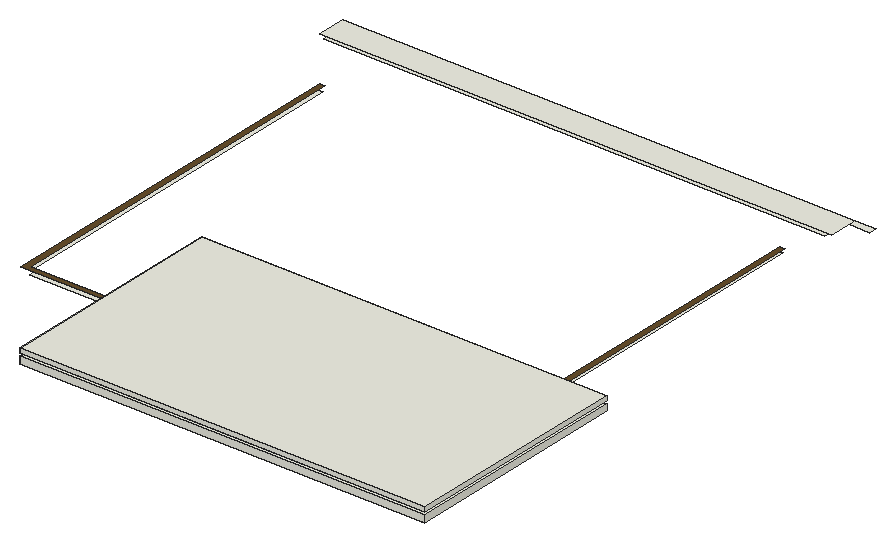
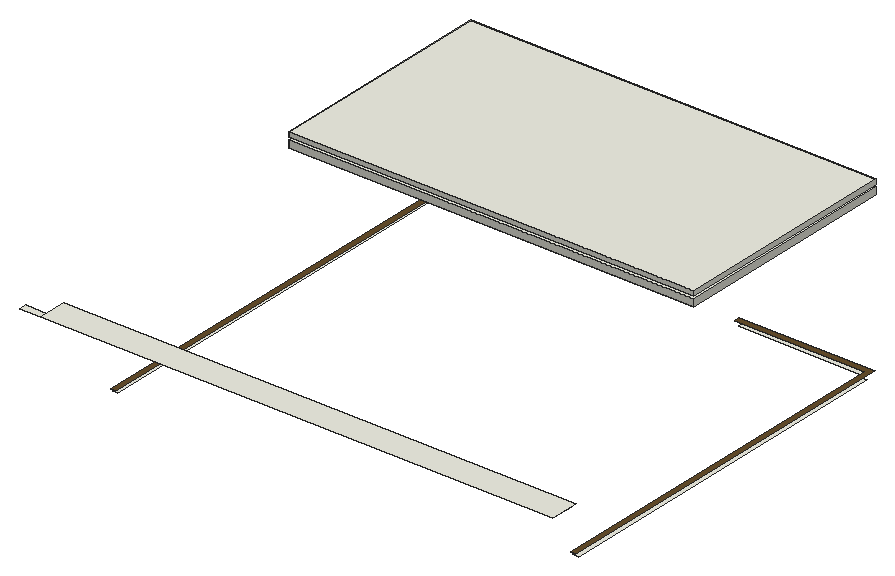
# SketchUp Ruby script. Lengths in inches.
U = 1.inch
M = Sketchup.active_model
def pt(a) = Geom::Point3d.new(a.map { |v| v * U })
def face(e, loops, mat)
  f = e.add_face(loops[0].map { |a| pt(a) })
  loops[1..].each { |l| e.add_face(l.map { |a| pt(a) }).erase! }
  f.material = f.back_material = mat if mat
  f
end
# faces: each face lists its corners as indices into pts; further lists are holes
def faces(e, pts, list, mat = nil) = list.each { |f| face(e, (f[0].is_a?(Array) ? f : [f]).map { |l| l.map { |i| pts[i] } }, mat) }
# xy, xz, yz: faces in a plane at the given z, y or x. An outline is a flat list of corners, or four numbers for a rectangle; further outlines are holes
def ring(l) = l.size == 4 ? [[l[0], l[1]], [l[2], l[1]], [l[2], l[3]], [l[0], l[3]]] : l.each_slice(2).to_a
def flat(e, list, mat, &to3) = list.each { |f| face(e, (f[0].is_a?(Array) ? f : [f]).map { |l| ring(l).map { |u, v| to3.(u, v) } }, mat) }
def xy(e, z, list, mat = nil) = flat(e, list, mat) { |x, y| [x, y, z] }
def xz(e, y, list, mat = nil) = flat(e, list, mat) { |x, z| [x, y, z] }
def yz(e, x, list, mat = nil) = flat(e, list, mat) { |y, z| [x, y, z] }
def lines(e, pts, list) = list.each { |a, b| e.add_line(pt(pts[a]), pt(pts[b])) }
# prism: a flat outline (further loops are holes) pulled along v
def prism(e, loops, v, mat = nil)
  f = face(e, loops, mat); d = Geom::Vector3d.new(v.map { |x| x * U })
  f.pushpull(f.normal.samedirection?(d) ? d.length : -d.length)
end
def box(e, o, s, mat = nil) = prism(e, [[o, [o[0] + s[0], o[1], o[2]], [o[0] + s[0], o[1] + s[1], o[2]], [o[0], o[1] + s[1], o[2]]]], [0, 0, s[2]], mat)
def at(x, y, z, deg = 0) = Geom::Transformation.translation(pt([x, y, z])) * Geom::Transformation.rotation(ORIGIN, Z_AXIS, deg.degrees)
def axes(o, x, y, z) = Geom::Transformation.new([*x, 0, *y, 0, *z, 0, *pt(o).to_a, 1])
def part(name) = M.definitions.add(name)
# library, detail: a bought-in or finely detailed component or shape, given as its bounding box
def library(name, o, s) = part(name).tap { |d| box(d.entities, o, s) }
def detail(e, o, s) = box(e.add_group.entities, o, s)
def put(e, d, t, mat = nil) = e.add_instance(d, t).tap { |i| i.material = mat if mat }
def group(e, t, mat = nil) = e.add_group.tap { |g| g.transformation = t; g.material = mat if mat }.entities
root = M.entities
M.materials.add("D01_Frost_White").color = [238, 238, 227]
M.materials.add("Wood_Veneer_15_1K").color = [103, 79, 44]
c1 = library("Sphere Light\#11",[-6.67,-6.67,-6.67],[13.34,13.34,13.34])
c2 = library("Sphere Light\#4",[-6.56,-6.56,-6.56],[13.12,13.12,13.12])
c3 = library("Sphere Light\#6",[-6.51,-6.51,-6.51],[13.02,13.02,13.02])
c4 = library("Sphere Light\#10",[-6.32,-6.32,-6.32],[12.64,12.64,12.64])
c5 = library("Sphere Light\#2",[-6.18,-6.18,-6.18],[12.36,12.36,12.36])
c6 = library("Sphere Light\#14",[-5.96,-5.96,-5.96],[11.92,11.92,11.92])
c7 = library("Sphere Light\#12",[-5.88,-5.88,-5.88],[11.76,11.76,11.76])
c8 = library("Sphere Light\#13",[-5.78,-5.78,-5.78],[11.56,11.56,11.56])
c9 = library("Sphere Light\#5",[-5.67,-5.67,-5.67],[11.34,11.34,11.34])
c10 = library("Sphere Light\#3",[-5.33,-5.33,-5.33],[10.66,10.66,10.66])
c11 = library("Sphere Light\#9",[-5.28,-5.28,-5.28],[10.56,10.56,10.56])
c12 = library("Sphere Light\#7",[-4.97,-4.97,-4.97],[9.94,9.94,9.94])
c13 = library("Sphere Light\#8",[-4.8125,-4.8125,-4.8125],[9.625,9.625,9.625])
xy(root,303,[[11.5,361,115,365.5],[4,368.5,8.5,673.01]],"D01_Frost_White")
xy(root,304,[[377.5,365.5,382,692]],"D01_Frost_White")
xy(root,306,[[4,361,118,361,118,365.5,8.5,365.5,8.5,676.01,4,676.01],[316,361,382,361,382,694,377.5,694,377.5,365.5,316,365.5]],"Wood_Veneer_15_1K")
xy(root,336,[[[118,217,460,409],[316,265,322,265,322,269,334,269,334,265,340,265,340,269,346,269,346,265,352,265,352,269,358,269,358,265,364,265,364,269,370,269,370,265,376,265,376,269,382,269,382,265,388,265,388,269,394,269,394,265,400,265,400,269,406,269,406,265,412,265,412,271,408,271,408,277,412,277,412,283,408,283,408,289,412,289,412,295,408,295,408,301,412,301,412,307,408,307,408,313,412,313,412,319,408,319,408,325,412,325,412,331,408,331,408,337,412,337,412,343,408,343,408,349,412,349,412,355,408,355,408,361,316,361,316,355,320,355,320,349,316,349,316,343,320,343,320,337,316,337,316,331,320,331,320,325,316,325,316,319,320,319,320,313,316,313,316,307,320,307,320,301,316,301,316,295,320,295,320,289,316,289,316,283,320,283,320,271,316,271],[142,373,166,385],[142,241,166,253],[448,271,449.55,271.2,451,271.8,452.24,272.76,453.2,274,453.8,275.45,454,277,453.8,278.55,453.2,280,452.24,281.24,451,282.2,449.55,282.8,448,283,446.45,282.8,445,282.2,443.76,281.24,442.8,280,442.2,278.55,442,277,442.2,275.45,442.8,274,443.76,272.76,445,271.8,446.45,271.2],[407,223,408.55,223.2,410,223.8,411.24,224.76,412.2,226,412.8,227.45,413,229,412.8,230.55,412.2,232,411.24,233.24,410,234.2,408.55,234.8,407,235,405.45,234.8,404,234.2,402.76,233.24,401.8,232,401.2,230.55,401,229,401.2,227.45,401.8,226,402.76,224.76,404,223.8,405.45,223.2],[448,307,449.55,307.2,451,307.8,452.24,308.76,453.2,310,453.8,311.45,454,313,453.8,314.55,453.2,316,452.24,317.24,451,318.2,449.55,318.8,448,319,446.45,318.8,445,318.2,443.76,317.24,442.8,316,442.2,314.55,442,313,442.2,311.45,442.8,310,443.76,308.76,445,307.8,446.45,307.2],[195,223,196.55,223.2,198,223.8,199.24,224.76,200.2,226,200.8,227.45,201,229,200.8,230.55,200.2,232,199.24,233.24,198,234.2,196.55,234.8,195,235,193.45,234.8,192,234.2,190.76,233.24,189.8,232,189.2,230.55,189,229,189.2,227.45,189.8,226,190.76,224.76,192,223.8,193.45,223.2],[248,223,249.55,223.2,251,223.8,252.24,224.76,253.2,226,253.8,227.45,254,229,253.8,230.55,253.2,232,252.24,233.24,251,234.2,249.55,234.8,248,235,246.45,234.8,245,234.2,243.76,233.24,242.8,232,242.2,230.55,242,229,242.2,227.45,242.8,226,243.76,224.76,245,223.8,246.45,223.2],[301,223,302.55,223.2,304,223.8,305.24,224.76,306.2,226,306.8,227.45,307,229,306.8,230.55,306.2,232,305.24,233.24,304,234.2,302.55,234.8,301,235,299.45,234.8,298,234.2,296.76,233.24,295.8,232,295.2,230.55,295,229,295.2,227.45,295.8,226,296.76,224.76,298,223.8,299.45,223.2],[354,223,355.55,223.2,357,223.8,358.24,224.76,359.2,226,359.8,227.45,360,229,359.8,230.55,359.2,232,358.24,233.24,357,234.2,355.55,234.8,354,235,352.45,234.8,351,234.2,349.76,233.24,348.8,232,348.2,230.55,348,229,348.2,227.45,348.8,226,349.76,224.76,351,223.8,352.45,223.2],[232,391,233.55,391.2,235,391.8,236.24,392.76,237.2,394,237.8,395.45,238,397,237.8,398.55,237.2,400,236.24,401.24,235,402.2,233.55,402.8,232,403,230.45,402.8,229,402.2,227.76,401.24,226.8,400,226.2,398.55,226,397,226.2,395.45,226.8,394,227.76,392.76,229,391.8,230.45,391.2],[403,391,404.55,391.2,406,391.8,407.24,392.76,408.2,394,408.8,395.45,409,397,408.8,398.55,408.2,400,407.24,401.24,406,402.2,404.55,402.8,403,403,401.45,402.8,400,402.2,398.76,401.24,397.8,400,397.2,398.55,397,397,397.2,395.45,397.8,394,398.76,392.76,400,391.8,401.45,391.2],[346,391,347.55,391.2,349,391.8,350.24,392.76,351.2,394,351.8,395.45,352,397,351.8,398.55,351.2,400,350.24,401.24,349,402.2,347.55,402.8,346,403,344.45,402.8,343,402.2,341.76,401.24,340.8,400,340.2,398.55,340,397,340.2,395.45,340.8,394,341.76,392.76,343,391.8,344.45,391.2],[289,391,290.55,391.2,292,391.8,293.24,392.76,294.2,394,294.8,395.45,295,397,294.8,398.55,294.2,400,293.24,401.24,292,402.2,290.55,402.8,289,403,287.45,402.8,286,402.2,284.76,401.24,283.8,400,283.2,398.55,283,397,283.2,395.45,283.8,394,284.76,392.76,286,391.8,287.45,391.2],[175,391,176.55,391.2,178,391.8,179.24,392.76,180.2,394,180.8,395.45,181,397,180.8,398.55,180.2,400,179.24,401.24,178,402.2,176.55,402.8,175,403,173.45,402.8,172,402.2,170.76,401.24,169.8,400,169.2,398.55,169,397,169.2,395.45,169.8,394,170.76,392.76,172,391.8,173.45,391.2],[448,343,449.55,343.2,451,343.8,452.24,344.76,453.2,346,453.8,347.45,454,349,453.8,350.55,453.2,352,452.24,353.24,451,354.2,449.55,354.8,448,355,446.45,354.8,445,354.2,443.76,353.24,442.8,352,442.2,350.55,442,349,442.2,347.45,442.8,346,443.76,344.76,445,343.8,446.45,343.2]],[316,265,322,265,322,269,334,269,334,265,340,265,340,269,346,269,346,265,352,265,352,269,358,269,358,265,364,265,364,269,370,269,370,265,376,265,376,269,382,269,382,265,388,265,388,269,394,269,394,265,400,265,400,269,406,269,406,265,412,265,412,271,316,271],[320,271,322,271,322,361,316,361,316,355,320,355,320,349,316,349,316,343,320,343,320,337,316,337,316,331,320,331,320,325,316,325,316,319,320,319,320,313,316,313,316,307,320,307,320,301,316,301,316,295,320,295,320,289,316,289,316,283,320,283],[322,271,406,355],[406,271,408,271,408,277,412,277,412,283,408,283,408,289,412,289,412,295,408,295,408,301,412,301,412,307,408,307,408,313,412,313,412,319,408,319,408,325,412,325,412,331,408,331,408,337,412,337,412,343,408,343,408,349,412,349,412,355,408,355,408,361,406,361],
  [322,355,406,361]],"D01_Frost_White")
xy(root,339,[[195,223,193.45,223.2,192,223.8,190.76,224.76,189.8,226,189.2,227.45,189,229,189.2,230.55,189.8,232,190.76,233.24,192,234.2,193.45,234.8,195,235,196.55,234.8,198,234.2,199.24,233.24,200.2,232,200.8,230.55,201,229,200.8,227.45,200.2,226,199.24,224.76,198,223.8,196.55,223.2],[248,223,246.45,223.2,245,223.8,243.76,224.76,242.8,226,242.2,227.45,242,229,242.2,230.55,242.8,232,243.76,233.24,245,234.2,246.45,234.8,248,235,249.55,234.8,251,234.2,252.24,233.24,253.2,232,253.8,230.55,254,229,253.8,227.45,253.2,226,252.24,224.76,251,223.8,249.55,223.2],[301,223,299.45,223.2,298,223.8,296.76,224.76,295.8,226,295.2,227.45,295,229,295.2,230.55,295.8,232,296.76,233.24,298,234.2,299.45,234.8,301,235,302.55,234.8,304,234.2,305.24,233.24,306.2,232,306.8,230.55,307,229,306.8,227.45,306.2,226,305.24,224.76,304,223.8,302.55,223.2],[354,223,352.45,223.2,351,223.8,349.76,224.76,348.8,226,348.2,227.45,348,229,348.2,230.55,348.8,232,349.76,233.24,351,234.2,352.45,234.8,354,235,355.55,234.8,357,234.2,358.24,233.24,359.2,232,359.8,230.55,360,229,359.8,227.45,359.2,226,358.24,224.76,357,223.8,355.55,223.2],[407,223,405.45,223.2,404,223.8,402.76,224.76,401.8,226,401.2,227.45,401,229,401.2,230.55,401.8,232,402.76,233.24,404,234.2,405.45,234.8,407,235,408.55,234.8,410,234.2,411.24,233.24,412.2,232,412.8,230.55,413,229,412.8,227.45,412.2,226,411.24,224.76,410,223.8,408.55,223.2],
  [448,271,446.45,271.2,445,271.8,443.76,272.76,442.8,274,442.2,275.45,442,277,442.2,278.55,442.8,280,443.76,281.24,445,282.2,446.45,282.8,448,283,449.55,282.8,451,282.2,452.24,281.24,453.2,280,453.8,278.55,454,277,453.8,275.45,453.2,274,452.24,272.76,451,271.8,449.55,271.2],[448,307,446.45,307.2,445,307.8,443.76,308.76,442.8,310,442.2,311.45,442,313,442.2,314.55,442.8,316,443.76,317.24,445,318.2,446.45,318.8,448,319,449.55,318.8,451,318.2,452.24,317.24,453.2,316,453.8,314.55,454,313,453.8,311.45,453.2,310,452.24,308.76,451,307.8,449.55,307.2],[448,343,446.45,343.2,445,343.8,443.76,344.76,442.8,346,442.2,347.45,442,349,442.2,350.55,442.8,352,443.76,353.24,445,354.2,446.45,354.8,448,355,449.55,354.8,451,354.2,452.24,353.24,453.2,352,453.8,350.55,454,349,453.8,347.45,453.2,346,452.24,344.76,451,343.8,449.55,343.2],[175,391,173.45,391.2,172,391.8,170.76,392.76,169.8,394,169.2,395.45,169,397,169.2,398.55,169.8,400,170.76,401.24,172,402.2,173.45,402.8,175,403,176.55,402.8,178,402.2,179.24,401.24,180.2,400,180.8,398.55,181,397,180.8,395.45,180.2,394,179.24,392.76,178,391.8,176.55,391.2],[232,391,230.45,391.2,229,391.8,227.76,392.76,226.8,394,226.2,395.45,226,397,226.2,398.55,226.8,400,227.76,401.24,229,402.2,230.45,402.8,232,403,233.55,402.8,235,402.2,236.24,401.24,237.2,400,237.8,398.55,238,397,237.8,395.45,237.2,394,236.24,392.76,235,391.8,233.55,391.2],
  [289,391,287.45,391.2,286,391.8,284.76,392.76,283.8,394,283.2,395.45,283,397,283.2,398.55,283.8,400,284.76,401.24,286,402.2,287.45,402.8,289,403,290.55,402.8,292,402.2,293.24,401.24,294.2,400,294.8,398.55,295,397,294.8,395.45,294.2,394,293.24,392.76,292,391.8,290.55,391.2],[346,391,344.45,391.2,343,391.8,341.76,392.76,340.8,394,340.2,395.45,340,397,340.2,398.55,340.8,400,341.76,401.24,343,402.2,344.45,402.8,346,403,347.55,402.8,349,402.2,350.24,401.24,351.2,400,351.8,398.55,352,397,351.8,395.45,351.2,394,350.24,392.76,349,391.8,347.55,391.2],[403,391,401.45,391.2,400,391.8,398.76,392.76,397.8,394,397.2,395.45,397,397,397.2,398.55,397.8,400,398.76,401.24,400,402.2,401.45,402.8,403,403,404.55,402.8,406,402.2,407.24,401.24,408.2,400,408.8,398.55,409,397,408.8,395.45,408.2,394,407.24,392.76,406,391.8,404.55,391.2]],"D01_Frost_White")
xy(root,341,[[7,676.01,430,694]],"D01_Frost_White")
xy(root,342,[[[118,217,460,409],[134,245,432,381]],[134,245,432,381]],"D01_Frost_White")
xy(root,344,[[118,217,118,409,460,409,460,217,296,217,296,245,432,245,432,381,134,381,134,245,296,245,296,217],[4,676.01,436,700],[436,694,454,700]],"D01_Frost_White")
xy(root,348,[[118,217,460,409]],"D01_Frost_White")
xz(root,217,[[118,336,460,342],[118,344,460,348]],"D01_Frost_White")
xz(root,245,[[134,342,432,344]],"D01_Frost_White")
xz(root,381,[[134,342,432,344]],"D01_Frost_White")
xz(root,409,[[118,336,460,342],[118,344,460,348]],"D01_Frost_White")
yz(root,118,[[217,336,409,342],[217,344,409,348]],"D01_Frost_White")
yz(root,134,[[245,342,381,344]],"D01_Frost_White")
yz(root,432,[[245,342,381,344]],"D01_Frost_White")
yz(root,460,[[217,336,409,342],[217,344,409,348]],"D01_Frost_White")
p = [[195,223,336],[193.45,223.2,336],[193.45,223.2,339],[195,223,339],[196.55,223.2,336],[196.55,223.2,339],
  [248,223,336],[246.45,223.2,336],[246.45,223.2,339],[248,223,339],[249.55,223.2,336],[249.55,223.2,339],
  [301,223,336],[299.45,223.2,336],[299.45,223.2,339],[301,223,339],[302.55,223.2,336],[302.55,223.2,339],
  [354,223,336],[352.45,223.2,336],[352.45,223.2,339],[354,223,339],[355.55,223.2,336],[355.55,223.2,339],
  [407,223,336],[405.45,223.2,336],[405.45,223.2,339],[407,223,339],[408.55,223.2,336],[408.55,223.2,339],
  [192,223.8,336],[192,223.8,339],[198,223.8,336],[198,223.8,339],[245,223.8,336],[245,223.8,339],
  [251,223.8,336],[251,223.8,339],[298,223.8,336],[298,223.8,339],[304,223.8,336],[304,223.8,339],
  [351,223.8,336],[351,223.8,339],[357,223.8,336],[357,223.8,339],[404,223.8,336],[404,223.8,339],
  [410,223.8,336],[410,223.8,339],[190.76,224.76,336],[190.76,224.76,339],[199.24,224.76,336],[199.24,224.76,339],
  [243.76,224.76,336],[243.76,224.76,339],[252.24,224.76,336],[252.24,224.76,339],[296.76,224.76,336],[296.76,224.76,339],
  [305.24,224.76,336],[305.24,224.76,339],[349.76,224.76,336],[349.76,224.76,339],[358.24,224.76,336],[358.24,224.76,339],
  [402.76,224.76,336],[402.76,224.76,339],[411.24,224.76,336],[411.24,224.76,339],[189.8,226,336],[189.8,226,339],
  [200.2,226,336],[200.2,226,339],[242.8,226,336],[242.8,226,339],[253.2,226,336],[253.2,226,339],
  [295.8,226,336],[295.8,226,339],[306.2,226,336],[306.2,226,339],[348.8,226,336],[348.8,226,339],
  [359.2,226,336],[359.2,226,339],[401.8,226,336],[401.8,226,339],[412.2,226,336],[412.2,226,339],
  [189.2,227.45,336],[189.2,227.45,339],[200.8,227.45,336],[200.8,227.45,339],[242.2,227.45,336],[242.2,227.45,339],
  [253.8,227.45,336],[253.8,227.45,339],[295.2,227.45,336],[295.2,227.45,339],[306.8,227.45,336],[306.8,227.45,339],
  [348.2,227.45,336],[348.2,227.45,339],[359.8,227.45,336],[359.8,227.45,339],[401.2,227.45,336],[401.2,227.45,339],
  [412.8,227.45,336],[412.8,227.45,339],[189,229,336],[189,229,339],[201,229,336],[201,229,339],
  [242,229,336],[242,229,339],[254,229,336],[254,229,339],[295,229,336],[295,229,339],
  [307,229,336],[307,229,339],[348,229,336],[348,229,339],[360,229,336],[360,229,339],
  [401,229,336],[401,229,339],[413,229,336],[413,229,339],[189.2,230.55,336],[189.2,230.55,339],
  [200.8,230.55,336],[200.8,230.55,339],[242.2,230.55,336],[242.2,230.55,339],[253.8,230.55,336],[253.8,230.55,339],
  [295.2,230.55,336],[295.2,230.55,339],[306.8,230.55,336],[306.8,230.55,339],[348.2,230.55,336],[348.2,230.55,339],
  [359.8,230.55,336],[359.8,230.55,339],[401.2,230.55,336],[401.2,230.55,339],[412.8,230.55,336],[412.8,230.55,339],
  [189.8,232,336],[189.8,232,339],[200.2,232,336],[200.2,232,339],[242.8,232,336],[242.8,232,339],
  [253.2,232,336],[253.2,232,339],[295.8,232,336],[295.8,232,339],[306.2,232,336],[306.2,232,339],
  [348.8,232,336],[348.8,232,339],[359.2,232,336],[359.2,232,339],[401.8,232,336],[401.8,232,339],
  [412.2,232,336],[412.2,232,339],[190.76,233.24,336],[190.76,233.24,339],[199.24,233.24,336],[199.24,233.24,339],
  [243.76,233.24,336],[243.76,233.24,339],[252.24,233.24,336],[252.24,233.24,339],[296.76,233.24,336],[296.76,233.24,339],
  [305.24,233.24,336],[305.24,233.24,339],[349.76,233.24,336],[349.76,233.24,339],[358.24,233.24,336],[358.24,233.24,339],
  [402.76,233.24,336],[402.76,233.24,339],[411.24,233.24,336],[411.24,233.24,339],[192,234.2,336],[192,234.2,339],
  [198,234.2,336],[198,234.2,339],[245,234.2,336],[245,234.2,339],[251,234.2,336],[251,234.2,339],
  [298,234.2,336],[298,234.2,339],[304,234.2,336],[304,234.2,339],[351,234.2,336],[351,234.2,339],
  [357,234.2,336],[357,234.2,339],[404,234.2,336],[404,234.2,339],[410,234.2,336],[410,234.2,339],
  [193.45,234.8,336],[193.45,234.8,339],[196.55,234.8,336],[196.55,234.8,339],[246.45,234.8,336],[246.45,234.8,339],
  [249.55,234.8,336],[249.55,234.8,339],[299.45,234.8,336],[299.45,234.8,339],[302.55,234.8,336],[302.55,234.8,339],
  [352.45,234.8,336],[352.45,234.8,339],[355.55,234.8,336],[355.55,234.8,339],[405.45,234.8,336],[405.45,234.8,339],
  [408.55,234.8,336],[408.55,234.8,339],[195,235,336],[195,235,339],[248,235,336],[248,235,339],
  [301,235,336],[301,235,339],[354,235,336],[354,235,339],[407,235,336],[407,235,339],
  [448,271,336],[446.45,271.2,336],[446.45,271.2,339],[448,271,339],[449.55,271.2,336],[449.55,271.2,339],
  [445,271.8,336],[445,271.8,339],[451,271.8,336],[451,271.8,339],[443.76,272.76,336],[443.76,272.76,339],
  [452.24,272.76,336],[452.24,272.76,339],[442.8,274,336],[442.8,274,339],[453.2,274,336],[453.2,274,339],
  [442.2,275.45,336],[442.2,275.45,339],[453.8,275.45,336],[453.8,275.45,339],[442,277,336],[442,277,339],
  [454,277,336],[454,277,339],[442.2,278.55,336],[442.2,278.55,339],[453.8,278.55,336],[453.8,278.55,339],
  [442.8,280,336],[442.8,280,339],[453.2,280,336],[453.2,280,339],[443.76,281.24,336],[443.76,281.24,339],
  [452.24,281.24,336],[452.24,281.24,339],[445,282.2,336],[445,282.2,339],[451,282.2,336],[451,282.2,339],
  [446.45,282.8,336],[446.45,282.8,339],[449.55,282.8,336],[449.55,282.8,339],[448,283,336],[448,283,339],
  [448,307,336],[446.45,307.2,336],[446.45,307.2,339],[448,307,339],[449.55,307.2,336],[449.55,307.2,339],
  [445,307.8,336],[445,307.8,339],[451,307.8,336],[451,307.8,339],[443.76,308.76,336],[443.76,308.76,339],
  [452.24,308.76,336],[452.24,308.76,339],[442.8,310,336],[442.8,310,339],[453.2,310,336],[453.2,310,339],
  [442.2,311.45,336],[442.2,311.45,339],[453.8,311.45,336],[453.8,311.45,339],[442,313,336],[442,313,339],
  [454,313,336],[454,313,339],[442.2,314.55,336],[442.2,314.55,339],[453.8,314.55,336],[453.8,314.55,339],
  [442.8,316,336],[442.8,316,339],[453.2,316,336],[453.2,316,339],[443.76,317.24,336],[443.76,317.24,339],
  [452.24,317.24,336],[452.24,317.24,339],[445,318.2,336],[445,318.2,339],[451,318.2,336],[451,318.2,339],
  [446.45,318.8,336],[446.45,318.8,339],[449.55,318.8,336],[449.55,318.8,339],[448,319,336],[448,319,339],
  [448,343,336],[446.45,343.2,336],[446.45,343.2,339],[448,343,339],[449.55,343.2,336],[449.55,343.2,339],
  [445,343.8,336],[445,343.8,339],[451,343.8,336],[451,343.8,339],[443.76,344.76,336],[443.76,344.76,339],
  [452.24,344.76,336],[452.24,344.76,339],[442.8,346,336],[442.8,346,339],[453.2,346,336],[453.2,346,339],
  [442.2,347.45,336],[442.2,347.45,339],[453.8,347.45,336],[453.8,347.45,339],[442,349,336],[442,349,339],
  [454,349,336],[454,349,339],[442.2,350.55,336],[442.2,350.55,339],[453.8,350.55,336],[453.8,350.55,339],
  [442.8,352,336],[442.8,352,339],[453.2,352,336],[453.2,352,339],[443.76,353.24,336],[443.76,353.24,339],
  [452.24,353.24,336],[452.24,353.24,339],[445,354.2,336],[445,354.2,339],[451,354.2,336],[451,354.2,339],
  [446.45,354.8,336],[446.45,354.8,339],[449.55,354.8,336],[449.55,354.8,339],[448,355,336],[448,355,339],
  [175,391,336],[173.45,391.2,336],[173.45,391.2,339],[175,391,339],[176.55,391.2,336],[176.55,391.2,339],
  [232,391,336],[230.45,391.2,336],[230.45,391.2,339],[232,391,339],[233.55,391.2,336],[233.55,391.2,339],
  [289,391,336],[287.45,391.2,336],[287.45,391.2,339],[289,391,339],[290.55,391.2,336],[290.55,391.2,339],
  [346,391,336],[344.45,391.2,336],[344.45,391.2,339],[346,391,339],[347.55,391.2,336],[347.55,391.2,339],
  [403,391,336],[401.45,391.2,336],[401.45,391.2,339],[403,391,339],[404.55,391.2,336],[404.55,391.2,339],
  [172,391.8,336],[172,391.8,339],[178,391.8,336],[178,391.8,339],[229,391.8,336],[229,391.8,339],
  [235,391.8,336],[235,391.8,339],[286,391.8,336],[286,391.8,339],[292,391.8,336],[292,391.8,339],
  [343,391.8,336],[343,391.8,339],[349,391.8,336],[349,391.8,339],[400,391.8,336],[400,391.8,339],
  [406,391.8,336],[406,391.8,339],[170.76,392.76,336],[170.76,392.76,339],[179.24,392.76,336],[179.24,392.76,339],
  [227.76,392.76,336],[227.76,392.76,339],[236.24,392.76,336],[236.24,392.76,339],[284.76,392.76,336],[284.76,392.76,339],
  [293.24,392.76,336],[293.24,392.76,339],[341.76,392.76,336],[341.76,392.76,339],[350.24,392.76,336],[350.24,392.76,339],
  [398.76,392.76,336],[398.76,392.76,339],[407.24,392.76,336],[407.24,392.76,339],[169.8,394,336],[169.8,394,339],
  [180.2,394,336],[180.2,394,339],[226.8,394,336],[226.8,394,339],[237.2,394,336],[237.2,394,339],
  [283.8,394,336],[283.8,394,339],[294.2,394,336],[294.2,394,339],[340.8,394,336],[340.8,394,339],
  [351.2,394,336],[351.2,394,339],[397.8,394,336],[397.8,394,339],[408.2,394,336],[408.2,394,339],
  [169.2,395.45,336],[169.2,395.45,339],[180.8,395.45,336],[180.8,395.45,339],[226.2,395.45,336],[226.2,395.45,339],
  [237.8,395.45,336],[237.8,395.45,339],[283.2,395.45,336],[283.2,395.45,339],[294.8,395.45,336],[294.8,395.45,339],
  [340.2,395.45,336],[340.2,395.45,339],[351.8,395.45,336],[351.8,395.45,339],[397.2,395.45,336],[397.2,395.45,339],
  [408.8,395.45,336],[408.8,395.45,339],[169,397,336],[169,397,339],[181,397,336],[181,397,339],
  [226,397,336],[226,397,339],[238,397,336],[238,397,339],[283,397,336],[283,397,339],
  [295,397,336],[295,397,339],[340,397,336],[340,397,339],[352,397,336],[352,397,339],
  [397,397,336],[397,397,339],[409,397,336],[409,397,339],[169.2,398.55,336],[169.2,398.55,339],
  [180.8,398.55,336],[180.8,398.55,339],[226.2,398.55,336],[226.2,398.55,339],[237.8,398.55,336],[237.8,398.55,339],
  [283.2,398.55,336],[283.2,398.55,339],[294.8,398.55,336],[294.8,398.55,339],[340.2,398.55,336],[340.2,398.55,339],
  [351.8,398.55,336],[351.8,398.55,339],[397.2,398.55,336],[397.2,398.55,339],[408.8,398.55,336],[408.8,398.55,339],
  [169.8,400,336],[169.8,400,339],[180.2,400,336],[180.2,400,339],[226.8,400,336],[226.8,400,339],
  [237.2,400,336],[237.2,400,339],[283.8,400,336],[283.8,400,339],[294.2,400,336],[294.2,400,339],
  [340.8,400,336],[340.8,400,339],[351.2,400,336],[351.2,400,339],[397.8,400,336],[397.8,400,339],
  [408.2,400,336],[408.2,400,339],[170.76,401.24,336],[170.76,401.24,339],[179.24,401.24,336],[179.24,401.24,339],
  [227.76,401.24,336],[227.76,401.24,339],[236.24,401.24,336],[236.24,401.24,339],[284.76,401.24,336],[284.76,401.24,339],
  [293.24,401.24,336],[293.24,401.24,339],[341.76,401.24,336],[341.76,401.24,339],[350.24,401.24,336],[350.24,401.24,339],
  [398.76,401.24,336],[398.76,401.24,339],[407.24,401.24,336],[407.24,401.24,339],[172,402.2,336],[172,402.2,339],
  [178,402.2,336],[178,402.2,339],[229,402.2,336],[229,402.2,339],[235,402.2,336],[235,402.2,339],
  [286,402.2,336],[286,402.2,339],[292,402.2,336],[292,402.2,339],[343,402.2,336],[343,402.2,339],
  [349,402.2,336],[349,402.2,339],[400,402.2,336],[400,402.2,339],[406,402.2,336],[406,402.2,339],
  [173.45,402.8,336],[173.45,402.8,339],[176.55,402.8,336],[176.55,402.8,339],[230.45,402.8,336],[230.45,402.8,339],
  [233.55,402.8,336],[233.55,402.8,339],[287.45,402.8,336],[287.45,402.8,339],[290.55,402.8,336],[290.55,402.8,339],
  [344.45,402.8,336],[344.45,402.8,339],[347.55,402.8,336],[347.55,402.8,339],[401.45,402.8,336],[401.45,402.8,339],
  [404.55,402.8,336],[404.55,402.8,339],[175,403,336],[175,403,339],[232,403,336],[232,403,339],
  [289,403,336],[289,403,339],[346,403,336],[346,403,339],[403,403,336],[403,403,339]]
faces(root,p,[[0,1,2,3],[4,0,3,5],[6,7,8,9],[10,6,9,11],[12,13,14,15],[16,12,15,17],[18,19,20,21],[22,18,21,23],
  [24,25,26,27],[28,24,27,29],[1,30,31,2],[32,4,5,33],[7,34,35,8],[36,10,11,37],[13,38,39,14],[40,16,17,41],
  [19,42,43,20],[44,22,23,45],[25,46,47,26],[48,28,29,49],[30,50,51,31],[52,32,33,53],[34,54,55,35],[56,36,37,57],
  [38,58,59,39],[60,40,41,61],[42,62,63,43],[64,44,45,65],[46,66,67,47],[68,48,49,69],[50,70,71,51],[72,52,53,73],
  [54,74,75,55],[76,56,57,77],[58,78,79,59],[80,60,61,81],[62,82,83,63],[84,64,65,85],[66,86,87,67],[88,68,69,89],
  [70,90,91,71],[92,72,73,93],[74,94,95,75],[96,76,77,97],[78,98,99,79],[100,80,81,101],[82,102,103,83],[104,84,85,105],
  [86,106,107,87],[108,88,89,109],[90,110,111,91],[112,92,93,113],[94,114,115,95],[116,96,97,117],[98,118,119,99],[120,100,101,121],
  [102,122,123,103],[124,104,105,125],[106,126,127,107],[128,108,109,129],[110,130,131,111],[132,112,113,133],[114,134,135,115],[136,116,117,137],
  [118,138,139,119],[140,120,121,141],[122,142,143,123],[144,124,125,145],[126,146,147,127],[148,128,129,149],[130,150,151,131],[152,132,133,153],
  [134,154,155,135],[156,136,137,157],[138,158,159,139],[160,140,141,161],[142,162,163,143],[164,144,145,165],[146,166,167,147],[168,148,149,169],
  [150,170,171,151],[172,152,153,173],[154,174,175,155],[176,156,157,177],[158,178,179,159],[180,160,161,181],[162,182,183,163],[184,164,165,185],
  [166,186,187,167],[188,168,169,189],[170,190,191,171],[192,172,173,193],[174,194,195,175],[196,176,177,197],[178,198,199,179],[200,180,181,201],
  [182,202,203,183],[204,184,185,205],[186,206,207,187],[208,188,189,209],[190,210,211,191],[212,192,193,213],[194,214,215,195],[216,196,197,217],
  [198,218,219,199],[220,200,201,221],[202,222,223,203],[224,204,205,225],[206,226,227,207],[228,208,209,229],[210,230,231,211],[230,212,213,231],
  [214,232,233,215],[232,216,217,233],[218,234,235,219],[234,220,221,235],[222,236,237,223],[236,224,225,237],[226,238,239,227],[238,228,229,239],
  [240,241,242,243],[244,240,243,245],[241,246,247,242],[248,244,245,249],[246,250,251,247],[252,248,249,253],[250,254,255,251],[256,252,253,257],
  [254,258,259,255],[260,256,257,261],[258,262,263,259],[264,260,261,265],[262,266,267,263],[268,264,265,269],[266,270,271,267],[272,268,269,273],
  [270,274,275,271],[276,272,273,277],[274,278,279,275],[280,276,277,281],[278,282,283,279],[284,280,281,285],[282,286,287,283],[286,284,285,287],
  [288,289,290,291],[292,288,291,293],[289,294,295,290],[296,292,293,297],[294,298,299,295],[300,296,297,301],[298,302,303,299],[304,300,301,305],
  [302,306,307,303],[308,304,305,309],[306,310,311,307],[312,308,309,313],[310,314,315,311],[316,312,313,317],[314,318,319,315],[320,316,317,321],
  [318,322,323,319],[324,320,321,325],[322,326,327,323],[328,324,325,329],[326,330,331,327],[332,328,329,333],[330,334,335,331],[334,332,333,335],
  [336,337,338,339],[340,336,339,341],[337,342,343,338],[344,340,341,345],[342,346,347,343],[348,344,345,349],[346,350,351,347],[352,348,349,353],
  [350,354,355,351],[356,352,353,357],[354,358,359,355],[360,356,357,361],[358,362,363,359],[364,360,361,365],[362,366,367,363],[368,364,365,369],
  [366,370,371,367],[372,368,369,373],[370,374,375,371],[376,372,373,377],[374,378,379,375],[380,376,377,381],[378,382,383,379],[382,380,381,383],
  [384,385,386,387],[388,384,387,389],[390,391,392,393],[394,390,393,395],[396,397,398,399],[400,396,399,401],[402,403,404,405],[406,402,405,407],
  [408,409,410,411],[412,408,411,413],[385,414,415,386],[416,388,389,417],[391,418,419,392],[420,394,395,421],[397,422,423,398],[424,400,401,425],
  [403,426,427,404],[428,406,407,429],[409,430,431,410],[432,412,413,433],[414,434,435,415],[436,416,417,437],[418,438,439,419],[440,420,421,441],
  [422,442,443,423],[444,424,425,445],[426,446,447,427],[448,428,429,449],[430,450,451,431],[452,432,433,453],[434,454,455,435],[456,436,437,457],
  [438,458,459,439],[460,440,441,461],[442,462,463,443],[464,444,445,465],[446,466,467,447],[468,448,449,469],[450,470,471,451],[472,452,453,473],
  [454,474,475,455],[476,456,457,477],[458,478,479,459],[480,460,461,481],[462,482,483,463],[484,464,465,485],[466,486,487,467],[488,468,469,489],
  [470,490,491,471],[492,472,473,493],[474,494,495,475],[496,476,477,497],[478,498,499,479],[500,480,481,501],[482,502,503,483],[504,484,485,505],
  [486,506,507,487],[508,488,489,509],[490,510,511,491],[512,492,493,513],[494,514,515,495],[516,496,497,517],[498,518,519,499],[520,500,501,521],
  [502,522,523,503],[524,504,505,525],[506,526,527,507],[528,508,509,529],[510,530,531,511],[532,512,513,533],[514,534,535,515],[536,516,517,537],
  [518,538,539,519],[540,520,521,541],[522,542,543,523],[544,524,525,545],[526,546,547,527],[548,528,529,549],[530,550,551,531],[552,532,533,553],
  [534,554,555,535],[556,536,537,557],[538,558,559,539],[560,540,541,561],[542,562,563,543],[564,544,545,565],[546,566,567,547],[568,548,549,569],
  [550,570,571,551],[572,552,553,573],[554,574,575,555],[576,556,557,577],[558,578,579,559],[580,560,561,581],[562,582,583,563],[584,564,565,585],
  [566,586,587,567],[588,568,569,589],[570,590,591,571],[592,572,573,593],[574,594,595,575],[596,576,577,597],[578,598,599,579],[600,580,581,601],
  [582,602,603,583],[604,584,585,605],[586,606,607,587],[608,588,589,609],[590,610,611,591],[612,592,593,613],[594,614,615,595],[614,596,597,615],
  [598,616,617,599],[616,600,601,617],[602,618,619,603],[618,604,605,619],[606,620,621,607],[620,608,609,621],[610,622,623,611],[622,612,613,623]],"D01_Frost_White")
put(root,c1,at(347.57,397.32,339),"D01_Frost_White")
put(root,c2,at(301.36,228.15,339),"D01_Frost_White")
put(root,c3,at(406.88,228.37,339),"D01_Frost_White")
put(root,c4,at(404.19,397.5,339),"D01_Frost_White")
put(root,c5,at(194.96,228.73,339),"D01_Frost_White")
put(root,c6,at(175.22,397.41,339),"D01_Frost_White")
put(root,c7,at(289.83,397.97,339),"D01_Frost_White")
put(root,c8,at(232.58,397.05,339),"D01_Frost_White")
put(root,c9,at(354.09,229.32,339),"D01_Frost_White")
put(root,c10,at(247.96,228.48,339),"D01_Frost_White")
put(root,c11,at(447.62,349.64,339),"D01_Frost_White")
put(root,c12,at(447.86,276.97,339),"D01_Frost_White")
put(root,c13,at(447.38,313.4375,339),"D01_Frost_White")
